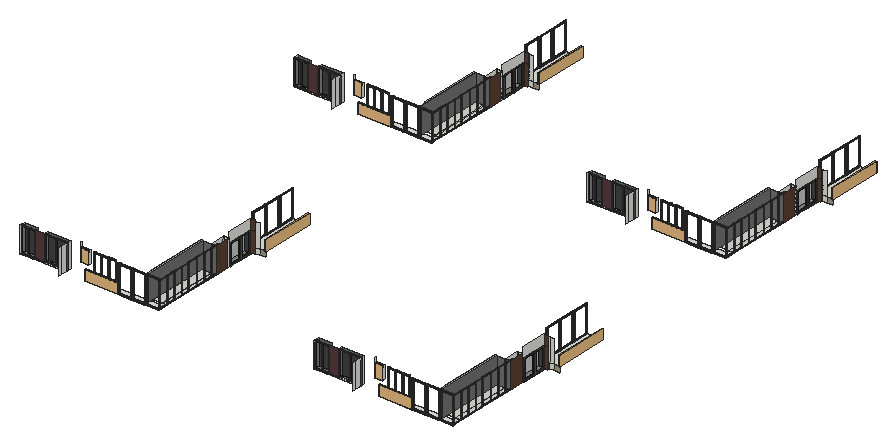
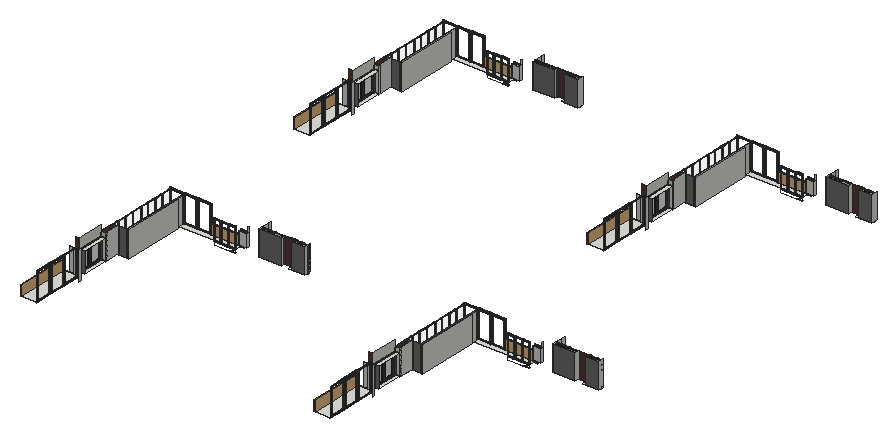
# SketchUp Ruby script. Lengths in inches.
U = 1.inch
M = Sketchup.active_model
def pt(a) = Geom::Point3d.new(a.map { |v| v * U })
def face(e, loops, mat)
  f = e.add_face(loops[0].map { |a| pt(a) })
  loops[1..].each { |l| e.add_face(l.map { |a| pt(a) }).erase! }
  f.material = f.back_material = mat if mat
  f
end
# faces: each face lists its corners as indices into pts; further lists are holes
def faces(e, pts, list, mat = nil) = list.each { |f| face(e, (f[0].is_a?(Array) ? f : [f]).map { |l| l.map { |i| pts[i] } }, mat) }
# xy, xz, yz: faces in a plane at the given z, y or x. An outline is a flat list of corners, or four numbers for a rectangle; further outlines are holes
def ring(l) = l.size == 4 ? [[l[0], l[1]], [l[2], l[1]], [l[2], l[3]], [l[0], l[3]]] : l.each_slice(2).to_a
def flat(e, list, mat, &to3) = list.each { |f| face(e, (f[0].is_a?(Array) ? f : [f]).map { |l| ring(l).map { |u, v| to3.(u, v) } }, mat) }
def xy(e, z, list, mat = nil) = flat(e, list, mat) { |x, y| [x, y, z] }
def xz(e, y, list, mat = nil) = flat(e, list, mat) { |x, z| [x, y, z] }
def yz(e, x, list, mat = nil) = flat(e, list, mat) { |y, z| [x, y, z] }
def lines(e, pts, list) = list.each { |a, b| e.add_line(pt(pts[a]), pt(pts[b])) }
# prism: a flat outline (further loops are holes) pulled along v
def prism(e, loops, v, mat = nil)
  f = face(e, loops, mat); d = Geom::Vector3d.new(v.map { |x| x * U })
  f.pushpull(f.normal.samedirection?(d) ? d.length : -d.length)
end
def box(e, o, s, mat = nil) = prism(e, [[o, [o[0] + s[0], o[1], o[2]], [o[0] + s[0], o[1] + s[1], o[2]], [o[0], o[1] + s[1], o[2]]]], [0, 0, s[2]], mat)
def at(x, y, z, deg = 0) = Geom::Transformation.translation(pt([x, y, z])) * Geom::Transformation.rotation(ORIGIN, Z_AXIS, deg.degrees)
def axes(o, x, y, z) = Geom::Transformation.new([*x, 0, *y, 0, *z, 0, *pt(o).to_a, 1])
def part(name) = M.definitions.add(name)
# library, detail: a bought-in or finely detailed component or shape, given as its bounding box
def library(name, o, s) = part(name).tap { |d| box(d.entities, o, s) }
def detail(e, o, s) = box(e.add_group.entities, o, s)
def put(e, d, t, mat = nil) = e.add_instance(d, t).tap { |i| i.material = mat if mat }
def group(e, t, mat = nil) = e.add_group.tap { |g| g.transformation = t; g.material = mat if mat }.entities
root = M.entities
M.materials.add("Glass_Tinted_Gray").color = [0, 0, 0]
M.materials["Glass_Tinted_Gray"].alpha = 0.125
M.materials.add("Glazing").color = [128, 128, 128]
M.materials["Glazing"].alpha = 0.05
M.materials.add("Powdercoating").color = [41, 44, 40]
M.materials.add("Wine2").color = [0, 0, 0]
M.materials["Wine2"].alpha = 0
M.materials.add("[0130_Gainsboro]").color = [39, 45, 50]
M.materials.add("[0135_DarkGray]").color = [81, 81, 81]
M.materials.add("[Color M05]").color = [114, 114, 114]
M.materials.add("[Color M06]").color = [86, 86, 86]
M.materials.add("[Concrete Tile]").color = [165, 155, 133]
M.materials.add("[Granite Brown]").color = [89, 59, 61]
M.materials.add("[Granite Brown]1").color = [89, 63, 50]
M.materials.add("[Mirror 02]").color = [229, 229, 229]
M.materials.add("[Terrazzo Light Blue]").color = [196, 214, 227]
c1 = part("Framed glazing panel")
xy(c1.entities,0,[[0,-0.98,43.07,0],[0,0,43.07,1.4]],"[0130_Gainsboro]")
xy(c1.entities,0.3,[[0.3,-1.43,42.77,-0.98]],"[0130_Gainsboro]")
xy(c1.entities,2.95,[[2.95,-1.43,40.12,-0.63],[2.95,-0.63,40.12,0],[2.95,0,40.12,0.64],[2.95,0.64,40.12,1.4]],"[0130_Gainsboro]")
xy(c1.entities,3.54,[[3.54,-0.63,39.53,0],[3.54,0,39.53,0.64]],"[0130_Gainsboro]")
xy(c1.entities,111.8125,[[3.54,-0.63,39.53,0],[3.54,0,39.53,0.64]],"[0130_Gainsboro]")
xy(c1.entities,112.4,[[2.95,-1.43,40.12,-0.63],[2.95,-0.63,40.12,0],[2.95,0,40.12,0.64],[2.95,0.64,40.12,1.4]],"[0130_Gainsboro]")
xy(c1.entities,115.05,[[0.3,-1.43,42.77,-0.98]],"[0130_Gainsboro]")
xy(c1.entities,115.35,[[0,-0.98,43.07,0],[0,0,43.07,1.4]],"[0130_Gainsboro]")
xz(c1.entities,-1.43,[[[0.3,0.3,42.77,115.05],[2.95,2.95,40.12,112.4]]],"[0130_Gainsboro]")
xz(c1.entities,-0.98,[[[0,0,43.07,115.35],[0.3,0.3,42.77,115.05]]],"[0130_Gainsboro]")
xz(c1.entities,-0.63,[[[2.95,2.95,40.12,112.4],[3.54,3.54,39.53,111.8125]]],"[0130_Gainsboro]")
xz(c1.entities,0,[[3.54,3.54,39.53,111.8125]],"Wine2")
xz(c1.entities,0,[[[0,0,43.07,115.35],[2.95,2.95,40.12,112.4]],[[2.95,2.95,40.12,112.4],[3.54,3.54,39.53,111.8125]]],"[0130_Gainsboro]")
xz(c1.entities,0.64,[[[2.95,2.95,40.12,112.4],[3.54,3.54,39.53,111.8125]]],"[0130_Gainsboro]")
xz(c1.entities,1.4,[[[0,0,43.07,115.35],[2.95,2.95,40.12,112.4]]],"[0130_Gainsboro]")
yz(c1.entities,0,[[-0.98,0,0,115.35],[0,0,1.4,115.35]],"[0130_Gainsboro]")
yz(c1.entities,0.3,[[-1.43,0.3,-0.98,115.05]],"[0130_Gainsboro]")
yz(c1.entities,2.95,[[-1.43,2.95,-0.63,112.4],[-0.63,2.95,0,112.4],[0,2.95,0.64,112.4],[0.64,2.95,1.4,112.4]],"[0130_Gainsboro]")
yz(c1.entities,3.54,[[-0.63,3.54,0,111.8125],[0,3.54,0.64,111.8125]],"[0130_Gainsboro]")
yz(c1.entities,39.53,[[-0.63,3.54,0,111.8125],[0,3.54,0.64,111.8125]],"[0130_Gainsboro]")
yz(c1.entities,40.12,[[-1.43,2.95,-0.63,112.4],[-0.63,2.95,0,112.4],[0,2.95,0.64,112.4],[0.64,2.95,1.4,112.4]],"[0130_Gainsboro]")
yz(c1.entities,42.77,[[-1.43,0.3,-0.98,115.05]],"[0130_Gainsboro]")
yz(c1.entities,43.07,[[-0.98,0,0,115.35],[0,0,1.4,115.35]],"[0130_Gainsboro]")
c2 = part("Glazed panel assembly")
put(c2.entities,c1,axes([90.57,1.43,0],[1.05148,0,0],[0,1,0],[0,0,1]))
put(c2.entities,c1,axes([0,1.43,0],[1.05148,0,0],[0,1,0],[0,0,1]))
put(c2.entities,c1,axes([45.29,1.43,0],[1.05148,0,0],[0,1,0],[0,0,1]))
c3 = library("Glass Railing",[0,0,0],[139.5,4.76,42])
c4 = part("PENTEK_RP Fineline 50S_Sliding_DoorCase_E1")
box(c4.entities,[0,0,0],[1.51,3.66,99.27],"[0135_DarkGray]")
c5 = part("PENTEK_RP Fineline 50S_SlidingDooe_Case_E2")
box(c5.entities,[0,0,0],[96.25,3.66,1.51],"[0135_DarkGray]")
c6 = part("pentek_RP Fineline 50S_SlidingDoor_Case")
put(c6.entities,c4,at(97.76,0,0))
put(c6.entities,c5,at(1.51,0,0))
put(c6.entities,c4,at(0,0,0))
put(c6.entities,c5,at(1.51,0,97.76))
c7 = part("PENTEK_RP Fineline 50S_SlidingDoor_GlazingBead_2")
box(c7.entities,[0,0,0],[0.56,0.59,94.39],"[0135_DarkGray]")
c8 = part("PENTEK_RP Fineline 50S_SlidingDoor_Glass")
box(c8.entities,[0,0,0],[46.58,0.16,94.39],"Glass_Tinted_Gray")
c9 = part("PENTEK_RP Fineline 50S_SlidingDoor_GlazingBead")
box(c9.entities,[0,0,0],[45.47,0.59,0.56],"[0135_DarkGray]")
c10 = part("PENTEK_RP Fineline 50S_SlidingDoor_Leaf_E1")
xy(c10.entities,0,[[0,0,0.93,1.97],[0.93,1.57,1.49,1.97]],"[0135_DarkGray]")
xy(c10.entities,96.25,[[0,0,0.93,0,0.93,1.57,1.49,1.57,1.49,1.97,0,1.97]],"[0135_DarkGray]")
xz(c10.entities,0,[[0,0,0.93,96.25]],"[0135_DarkGray]")
xz(c10.entities,1.57,[[0.93,0,1.49,95.32],[0.93,95.32,1.49,96.25]],"[0135_DarkGray]")
xz(c10.entities,1.97,[[0,0,1.49,96.25]],"[0135_DarkGray]")
yz(c10.entities,0,[[0,0,1.97,96.25]],"[0135_DarkGray]")
yz(c10.entities,0.93,[[0,0,1.57,0.93],[0,0.93,1.57,95.32],[0,95.32,1.57,96.25]],"[0135_DarkGray]")
yz(c10.entities,1.49,[[1.57,0,1.97,95.32],[1.57,95.32,1.97,96.25]],"[0135_DarkGray]")
c11 = part("PENTEK_RP Fineline 50S_SlidingDoor_Leaf_E2")
xy(c11.entities,0,[[0,0,0,1.57,0.56,1.57,0.56,1.97,46.02,1.97,46.02,1.57,46.58,1.57,46.58,0]],"[0135_DarkGray]")
xy(c11.entities,0.93,[[0,0,46.58,1.57]],"[0135_DarkGray]")
xy(c11.entities,1.49,[[0.56,1.57,46.02,1.97]],"[0135_DarkGray]")
xz(c11.entities,0,[[0,0,46.58,0.93]],"[0135_DarkGray]")
xz(c11.entities,1.57,[[0,0,0.56,0.93],[46.02,0,46.58,0.93],[0.56,0.93,46.02,1.49]],"[0135_DarkGray]")
xz(c11.entities,1.97,[[0.56,0,46.02,1.49]],"[0135_DarkGray]")
yz(c11.entities,0,[[0,0,1.57,0.93]],"[0135_DarkGray]")
yz(c11.entities,0.56,[[1.57,0,1.97,0.93],[1.57,0.93,1.97,1.49]],"[0135_DarkGray]")
yz(c11.entities,46.02,[[1.57,0,1.97,0.93],[1.57,0.93,1.97,1.49]],"[0135_DarkGray]")
yz(c11.entities,46.58,[[0,0,1.57,0.93]],"[0135_DarkGray]")
c12 = part("PENTEK_RP Fineline S_SlidingDoor_Leaf1")
put(c12.entities,c7,at(0.93,0,0.93))
put(c12.entities,c7,at(46.96,0,0.93))
put(c12.entities,c8,at(1.49,1.42,0.93))
put(c12.entities,c9,at(1.49,0,0.93))
put(c12.entities,c8,at(1.49,0.59,0.93),"[Terrazzo Light Blue]")
put(c12.entities,c10,at(0,0,0))
put(c12.entities,c10,axes([48.44,0,0],[-1,0,0],[0,1,0],[0,0,1]))
put(c12.entities,c11,axes([0.93,0,96.25],[1,0,0],[0,1,0],[0,0,-1]))
put(c12.entities,c11,at(0.93,0,0))
put(c12.entities,c9,at(1.49,0,94.77))
c13 = part("PENTEK_RP Fineline 50S_SlidingDoor_Leaf2")
put(c13.entities,c8,at(1.49,1.42,0.93))
put(c13.entities,c9,at(1.49,0,94.77))
put(c13.entities,c7,at(46.96,0,0.93))
put(c13.entities,c8,at(1.49,0.59,0.93),"[Mirror 02]")
put(c13.entities,c7,at(0.93,0,0.93))
put(c13.entities,c10,at(0,0,0))
put(c13.entities,c10,axes([48.44,0,0],[-1,0,0],[0,1,0],[0,0,1]))
put(c13.entities,c9,at(1.49,0,0.93))
put(c13.entities,c11,axes([0.93,0,96.25],[1,0,0],[0,1,0],[0,0,-1]))
put(c13.entities,c11,at(0.93,0,0))
c14 = part("PENTEK - Slimmest Steel Sliding Door / Window\#1")
put(c14.entities,c6,at(0,-1.88,-0.09))
put(c14.entities,c12,at(1.51,-2.27,1.42))
put(c14.entities,c13,at(49.32,-0.3,1.42))
c15 = part("Group\#15")
xy(c15.entities,0,[[0,-55.94,0.71,45.94]])
xy(c15.entities,0.2,[[0,-55.94,0.47,45.94],[0.47,45.94,0.71,46.42]])
xy(c15.entities,2.36,[[0.47,-55.94,0.71,46.42]])
xz(c15.entities,-55.94,[[0,0,0.71,0,0.71,2.36,0.47,2.36,0.47,0.2,0,0.2]])
xz(c15.entities,45.94,[[0,0,0.71,0.2]])
xz(c15.entities,46.42,[[0.47,0.2,0.71,2.36]])
yz(c15.entities,0,[[-55.94,0,45.94,0.2]])
yz(c15.entities,0.47,[[-55.94,0.2,46.42,2.36]])
yz(c15.entities,0.71,[[-55.94,0,45.94,0,45.94,0.2,46.42,0.2,46.42,2.36,-55.94,2.36]])
c16 = part("Group\#7")
xy(c16.entities,0,[[0,-59.09,0.71,45.94]])
xy(c16.entities,0.2,[[0,-59.09,0.47,45.94],[0.47,45.94,0.71,46.42]])
xy(c16.entities,2.36,[[0.47,-59.09,0.71,46.42]])
xz(c16.entities,-59.09,[[0,0,0.71,0,0.71,2.36,0.47,2.36,0.47,0.2,0,0.2]])
xz(c16.entities,45.94,[[0,0,0.71,0.2]])
xz(c16.entities,46.42,[[0.47,0.2,0.71,2.36]])
yz(c16.entities,0,[[-59.09,0,45.94,0.2]])
yz(c16.entities,0.47,[[-59.09,0.2,46.42,2.36]])
yz(c16.entities,0.71,[[-59.09,0,45.94,0,45.94,0.2,46.42,0.2,46.42,2.36,-59.09,2.36]])
c17 = part("Group\#16")
prism(c17.entities,[[[0.47,-56.18,0.2],[0,-56.18,0.2],[0,-56.18,0],[0.71,-56.18,0],[0.71,-56.18,2.36],[0.47,-56.18,2.36]]],[0,28.68,0])
c18 = part("Group\#10")
box(c18.entities,[-0.73,0,0],[27.99,0.55,102.05])
c19 = part("Group\#18")
xy(c19.entities,0,[[0.47,-56.18,0.47,-55.47,0,-55.47,0,-28.21,1.18,-28.21,1.18,-56.18]])
xy(c19.entities,0.2,[[0.71,-56.18,1.18,-28.21],[0,-55.47,0.47,-28.21],[0.47,-28.21,0.71,-27.74]])
xy(c19.entities,2.36,[[0.47,-56.18,0.71,-27.74]])
xz(c19.entities,-56.18,[[0.47,0,1.18,0,1.18,0.2,0.71,0.2,0.71,2.36,0.47,2.36]])
xz(c19.entities,-55.47,[[0,0,0.47,0.2]])
xz(c19.entities,-28.21,[[0,0,1.18,0.2]])
xz(c19.entities,-27.74,[[0.47,0.2,0.71,2.36]])
yz(c19.entities,0,[[-55.47,0,-28.21,0.2]])
yz(c19.entities,0.47,[[-56.18,0,-55.47,0.2],[-56.18,0.2,-27.74,2.36]])
yz(c19.entities,0.71,[[-56.18,0.2,-27.74,2.36]])
yz(c19.entities,1.18,[[-56.18,0,-28.21,0.2]])
c20 = part("Group\#34")
xy(c20.entities,0,[[-20.45,0,7.76,1.22]])
xy(c20.entities,0.06,[[-20.39,0.06,7.7,1.22]])
xy(c20.entities,0.47,[[-19.98,0,7.28,0.06]])
xy(c20.entities,101.89,[[-19.98,0,7.28,0.06]])
xy(c20.entities,102.3,[[-20.39,0.06,7.7,1.22]])
xy(c20.entities,102.36,[[-20.45,0,7.76,1.22]])
xz(c20.entities,0,[[[-20.45,0,7.76,102.36],[-19.98,0.47,7.28,101.89]]])
xz(c20.entities,0.06,[[[-20.39,0.06,7.7,102.3],[-19.98,0.47,7.28,101.89]]])
xz(c20.entities,1.22,[[[-20.45,0,7.76,102.36],[-20.39,0.06,7.7,102.3]]])
yz(c20.entities,-20.45,[[0,0,1.22,102.36]])
yz(c20.entities,-20.39,[[0.06,0.06,1.22,102.3]])
yz(c20.entities,-19.98,[[0,0.47,0.06,101.89]])
yz(c20.entities,7.28,[[0,0.47,0.06,101.89]])
yz(c20.entities,7.7,[[0.06,0.06,1.22,102.3]])
yz(c20.entities,7.76,[[0,0,1.22,102.36]])
c21 = part("Group\#6")
put(c21.entities,c15,axes([27.97,0,7.875],[1,0,0],[0,0,-1],[0,1,0]),"Powdercoating")
put(c21.entities,c16,axes([0.71,0,6.8],[-1,0,0],[0,0,-0.97687],[0,1,0]),"Powdercoating")
put(c21.entities,c17,axes([-27.5,0,-38.07],[0,0,-1],[-1,0,0],[0,1,0]),"Powdercoating")
put(c21.entities,c18,at(1.12,0.35,-38.39),"Glazing")
put(c21.entities,c19,axes([-27.5,0,63.35],[0,0,1],[-1,0,0],[0,1,0]),"Powdercoating")
put(c21.entities,c20,at(20.6875,1.0625,-38.54),"Powdercoating")
c22 = part("Sliding door assembly")
put(c22.entities,c21,at(-1.18,4.5,38.86))
g1 = group(c22.entities,at(84.74,4.5,38.86))
put(g1,c15,axes([-27.97,0,7.875],[-1,0,0],[0,0,-1],[0,1,0]),"Powdercoating")
put(g1,c16,axes([-0.71,0,6.8],[1,0,0],[0,0,-0.97687],[0,1,0]),"Powdercoating")
put(g1,c17,axes([27.5,0,-38.07],[0,0,-1],[1,0,0],[0,1,0]),"Powdercoating")
put(g1,c18,axes([-1.12,0.35,-38.39],[-1,0,0],[0,1,0],[0,0,1]),"Glazing")
put(g1,c19,axes([27.5,0,63.35],[0,0,1],[1,0,0],[0,1,0]),"Powdercoating")
put(g1,c20,axes([-20.6875,1.0625,-38.54],[-1,0,0],[0,1,0],[0,0,1]),"Powdercoating")
g2 = group(c22.entities,at(56.0625,4.5,38.86))
put(g2,c15,axes([-27.97,0,7.875],[-1,0,0],[0,0,-1],[0,1,0]),"Powdercoating")
put(g2,c17,axes([27.5,0,-38.07],[0,0,-1],[1,0,0],[0,1,0]),"Powdercoating")
put(g2,c18,axes([-1.12,0.35,-38.39],[-1,0,0],[0,1,0],[0,0,1]),"Glazing")
put(g2,c19,axes([27.5,0,63.35],[0,0,1],[1,0,0],[0,1,0]),"Powdercoating")
put(g2,c20,axes([-20.6875,1.0625,-38.54],[-1,0,0],[0,1,0],[0,0,1]),"Powdercoating")
g3 = group(g2,at(-0.71,0,6.8),"Powdercoating")
xy(g3,-45.34,[[0.47,0.2,0.71,2.36]])
xy(g3,-44.88,[[0,0,0.71,0.2]])
xy(g3,57.73,[[0,0,0.71,0,0.71,2.36,0.47,2.36,0.47,0.2,0,0.2]])
xz(g3,0,[[0,-44.88,0.71,57.73]])
xz(g3,0.2,[[0.47,-45.34,0.71,-44.88],[0,-44.88,0.47,57.73]])
xz(g3,2.36,[[0.47,-45.34,0.71,57.73]])
yz(g3,0,[[0,-44.88,0.2,57.73]])
yz(g3,0.47,[[0.2,-45.34,2.36,57.73]])
yz(g3,0.71,[[0.2,-45.34,2.36,-45.34,2.36,57.73,0,57.73,0,-44.88,0.2,-44.88]])
put(c22.entities,c21,axes([-33.94,4.5,38.86],[1.14218,0,0],[0,1,0],[0,0,1]))
c23 = part("sliding door")
put(c23.entities,c22,at(0,-4.5,-0.08))
c24 = library("Klein+raam",[128.36,12.7,0],[19.68,5.51,55.12])
xy(root,641.5625,[[611.65,1835.1875,632.49,1837.0625],[1829.84,1835.1875,1850.67,1837.0625],[611.65,3249.875,632.49,3251.75],[1829.84,3249.875,1850.67,3251.75]])
xy(root,641.875,[[611.65,1835.1875,632.49,1837.0625],[1829.84,1835.1875,1850.67,1837.0625],[611.65,3249.875,632.49,3251.75],[1829.84,3249.875,1850.67,3251.75]])
xy(root,648.6875,[[745.8,1795.6875,913.875,1795.6875,913.875,1833.5,890.875,1833.5,890.875,1822.9375,857.6875,1822.9375,857.6875,1812.1875,852.25,1812.1875,852.25,1822.9375,616.54,1822.9375,616.54,1799.9375,745.8,1799.9375],[1963.98,1795.6875,2132.0625,1795.6875,2132.0625,1833.5,2109.0625,1833.5,2109.0625,1822.9375,2075.875,1822.9375,2075.875,1812.1875,2070.4375,1812.1875,2070.4375,1822.9375,1834.73,1822.9375,1834.73,1799.9375,1963.98,1799.9375],[852.25,1812.1875,857.6875,1822.9375],[2070.4375,1812.1875,2075.875,1822.9375],[852.25,1822.9375,857.6875,1837.0625],
  [2070.4375,1822.9375,2075.875,1837.0625],[890.875,1833.5,913.875,1835.1875],[2109.0625,1833.5,2132.0625,1835.1875],[890.875,1835.1875,894.3125,2091.0625],[894.3125,1835.1875,913.875,2091.0625],
  [2109.0625,1835.1875,2112.5,2091.0625],[2112.5,1835.1875,2132.0625,2091.0625],[847.6875,1837.0625,852.25,2091.0625],[852.25,1837.0625,857.6875,2091.0625],[857.6875,1837.0625,890.875,2091.0625],
  [2065.875,1837.0625,2070.4375,2091.0625],[2070.4375,1837.0625,2075.875,2091.0625],[2075.875,1837.0625,2109.0625,2091.0625],[894.3125,2091.0625,913.875,2156.01],[2112.5,2091.0625,2132.0625,2156.01],
  [745.8,3210.375,913.875,3210.375,913.875,3248.1875,890.875,3248.1875,890.875,3237.625,857.6875,3237.625,857.6875,3226.875,852.25,3226.875,852.25,3237.625,616.54,3237.625,616.54,3214.625,745.8,3214.625],[1963.98,3210.375,2132.0625,3210.375,2132.0625,3248.1875,2109.0625,3248.1875,2109.0625,3237.625,2075.875,3237.625,2075.875,3226.875,2070.4375,3226.875,2070.4375,3237.625,1834.73,3237.625,1834.73,3214.625,1963.98,3214.625],[852.25,3226.875,857.6875,3237.625],[2070.4375,3226.875,2075.875,3237.625],[852.25,3237.625,857.6875,3251.75],
  [2070.4375,3237.625,2075.875,3251.75],[890.875,3248.1875,913.875,3249.875],[2109.0625,3248.1875,2132.0625,3249.875],[890.875,3249.875,894.3125,3505.75],[894.3125,3249.875,913.875,3505.75],
  [2109.0625,3249.875,2112.5,3505.75],[2112.5,3249.875,2132.0625,3505.75],[847.6875,3251.75,852.25,3505.75],[852.25,3251.75,857.6875,3505.75],[857.6875,3251.75,890.875,3505.75],
  [2065.875,3251.75,2070.4375,3505.75],[2070.4375,3251.75,2075.875,3505.75],[2075.875,3251.75,2109.0625,3505.75],[894.3125,3505.75,913.875,3570.7],[2112.5,3505.75,2132.0625,3570.7]])
xy(root,651.4375,[[333.89,1799.9375,401.8,1822.9375],[401.8,1799.9375,431.33,1806.5625],[431.33,1799.9375,523.04,1822.9375],[1552.08,1799.9375,1619.99,1822.9375],[1619.99,1799.9375,1649.52,1806.5625],
  [1649.52,1799.9375,1741.23,1822.9375],[333.89,3214.625,401.8,3237.625],[401.8,3214.625,431.33,3221.25],[431.33,3214.625,523.04,3237.625],[1552.08,3214.625,1619.99,3237.625],
  [1619.99,3214.625,1649.52,3221.25],[1649.52,3214.625,1741.23,3237.625]])
xy(root,653.36,[[890.875,2156.01,913.875,2266.33],[2109.0625,2156.01,2132.0625,2266.33],[890.875,3570.7,913.875,3681.01],[2109.0625,3570.7,2132.0625,3681.01]])
xy(root,660.0625,[[890.875,2295.875,954.6875,2518.89],[2109.0625,2295.875,2172.875,2518.89],[890.875,3710.5625,954.6875,3933.57],[2109.0625,3710.5625,2172.875,3933.57]])
xy(root,682.81,[[557.4,1837.0625,589.71,1845.8125],[1775.59,1837.0625,1807.9,1845.8125],[557.4,3251.75,589.71,3260.5],[1775.59,3251.75,1807.9,3260.5]])
xy(root,735.09,[[557.4,1837.0625,589.71,1845.8125],[1775.59,1837.0625,1807.9,1845.8125],[557.4,3251.75,589.71,3260.5],[1775.59,3251.75,1807.9,3260.5]])
xy(root,739.04,[[890.875,2156.01,913.875,2266.33],[2109.0625,2156.01,2132.0625,2266.33],[890.875,3570.7,913.875,3681.01],[2109.0625,3570.7,2132.0625,3681.01]])
xz(root,1806.5625,[[401.8,651.4375,431.33,651.4375,431.33,756,402.4,756,387.59,756.07,387.07,651.51],[1619.99,651.4375,1649.52,651.4375,1649.52,756,1620.59,756,1605.78,756.07,1605.26,651.51]],"[Granite Brown]")
xz(root,1812.1875,[[852.25,648.6875,857.6875,756],[2070.4375,648.6875,2075.875,756]])
xz(root,1822.9375,[[333.89,651.4375,387.07,651.4375,387.59,756,333.89,756],[431.33,651.4375,523.04,756],[1552.08,651.4375,1605.26,651.4375,1605.78,756,1552.08,756],[1649.52,651.4375,1741.23,756]],"[Color M05]")
xz(root,1835.1875,[[611.65,641.5625,632.49,641.875],[1829.84,641.5625,1850.67,641.875]])
xz(root,1835.1875,[[557.4,682.81,557.88,735.09],[1775.59,682.81,1776.07,735.09],[557.4,735.09,557.88,756],[1775.59,735.09,1776.07,756]],"[Granite Brown]")
xz(root,1845.8125,[[557.4,682.81,589.71,735.09],[1775.59,682.81,1807.9,735.09]])
xz(root,2091.0625,[[847.6875,648.6875,852.25,756],[852.25,648.6875,857.6875,756],[890.875,648.6875,894.3125,756],[2065.875,648.6875,2070.4375,756],[2070.4375,648.6875,2075.875,756],
  [2109.0625,648.6875,2112.5,756]])
xz(root,2091.0625,[[857.6875,648.6875,890.875,756],[894.3125,648.6875,913.875,756],[2075.875,648.6875,2109.0625,756],[2112.5,648.6875,2132.0625,756]],"[Color M05]")
xz(root,2156.01,[[894.3125,648.6875,913.875,653.36],[2112.5,648.6875,2132.0625,653.36],[890.875,653.36,894.3125,739.04],[894.3125,653.36,913.875,739.04],[2109.0625,653.36,2112.5,739.04],
  [2112.5,653.36,2132.0625,739.04],[894.3125,739.04,913.875,756],[2112.5,739.04,2132.0625,756]])
xz(root,2266.33,[[890.875,653.36,913.875,739.04],[2109.0625,653.36,2132.0625,739.04]],"[Color M05]")
xz(root,2266.33,[[913.875,653.36,930.75,739.04],[2132.0625,653.36,2148.9375,739.04],[913.875,739.04,930.75,779.36],[2132.0625,739.04,2148.9375,779.36]],"[Granite Brown]1")
xz(root,2295.875,[[913.875,637.75,930.75,660.0625],[2132.0625,637.75,2148.9375,660.0625],[890.875,660.0625,913.875,756],[913.875,660.0625,930.75,756],[2109.0625,660.0625,2132.0625,756],
  [2132.0625,660.0625,2148.9375,756]])
xz(root,2295.875,[[930.75,637.75,954.6875,660.0625],[2148.9375,637.75,2172.875,660.0625]],"[Concrete Tile]")
xz(root,3221.25,[[401.8,651.4375,431.33,651.4375,431.33,756,402.4,756,387.59,756.07,387.07,651.51],[1619.99,651.4375,1649.52,651.4375,1649.52,756,1620.59,756,1605.78,756.07,1605.26,651.51]],"[Granite Brown]")
xz(root,3226.875,[[852.25,648.6875,857.6875,756],[2070.4375,648.6875,2075.875,756]])
xz(root,3237.625,[[333.89,651.4375,387.07,651.4375,387.59,756,333.89,756],[431.33,651.4375,523.04,756],[1552.08,651.4375,1605.26,651.4375,1605.78,756,1552.08,756],[1649.52,651.4375,1741.23,756]],"[Color M05]")
xz(root,3249.875,[[611.65,641.5625,632.49,641.875],[1829.84,641.5625,1850.67,641.875]])
xz(root,3249.875,[[557.4,682.81,557.88,735.09],[1775.59,682.81,1776.07,735.09],[557.4,735.09,557.88,756],[1775.59,735.09,1776.07,756]],"[Granite Brown]")
xz(root,3260.5,[[557.4,682.81,589.71,735.09],[1775.59,682.81,1807.9,735.09]])
xz(root,3505.75,[[847.6875,648.6875,852.25,756],[852.25,648.6875,857.6875,756],[890.875,648.6875,894.3125,756],[2065.875,648.6875,2070.4375,756],[2070.4375,648.6875,2075.875,756],
  [2109.0625,648.6875,2112.5,756]])
xz(root,3505.75,[[857.6875,648.6875,890.875,756],[894.3125,648.6875,913.875,756],[2075.875,648.6875,2109.0625,756],[2112.5,648.6875,2132.0625,756]],"[Color M05]")
xz(root,3570.7,[[894.3125,648.6875,913.875,653.36],[2112.5,648.6875,2132.0625,653.36],[890.875,653.36,894.3125,739.04],[894.3125,653.36,913.875,739.04],[2109.0625,653.36,2112.5,739.04],
  [2112.5,653.36,2132.0625,739.04],[894.3125,739.04,913.875,756],[2112.5,739.04,2132.0625,756]])
xz(root,3681.01,[[890.875,653.36,913.875,739.04],[2109.0625,653.36,2132.0625,739.04]],"[Color M05]")
xz(root,3681.01,[[913.875,653.36,930.75,739.04],[2132.0625,653.36,2148.9375,739.04],[913.875,739.04,930.75,779.36],[2132.0625,739.04,2148.9375,779.36]],"[Granite Brown]1")
xz(root,3710.5625,[[913.875,637.75,930.75,660.0625],[2132.0625,637.75,2148.9375,660.0625],[890.875,660.0625,913.875,756],[913.875,660.0625,930.75,756],[2109.0625,660.0625,2132.0625,756],
  [2132.0625,660.0625,2148.9375,756]])
xz(root,3710.5625,[[930.75,637.75,954.6875,660.0625],[2148.9375,637.75,2172.875,660.0625]],"[Concrete Tile]")
yz(root,333.89,[[1799.9375,651.4375,1822.9375,756],[3214.625,651.4375,3237.625,756]])
yz(root,431.33,[[1806.5625,651.4375,1822.9375,756],[3221.25,651.4375,3237.625,756]])
yz(root,523.04,[[1763.25,651.4375,1822.9375,756],[3177.9375,651.4375,3237.625,756]])
yz(root,557.4,[[1835.1875,682.81,1845.8125,735.09],[3249.875,682.81,3260.5,735.09],[1835.1875,735.09,1837.0625,756],[3249.875,735.09,3251.75,756]])
yz(root,589.71,[[1837.0625,682.81,1845.8125,735.09],[3251.75,682.81,3260.5,735.09]])
yz(root,611.65,[[1835.1875,641.5625,1837.0625,641.875],[3249.875,641.5625,3251.75,641.875]])
yz(root,632.49,[[1835.1875,641.5625,1837.0625,641.875],[3249.875,641.5625,3251.75,641.875]])
yz(root,847.6875,[[1837.0625,648.6875,2091.0625,756],[3251.75,648.6875,3505.75,756]])
yz(root,852.25,[[1812.1875,648.6875,2091.0625,756],[3226.875,648.6875,3505.75,756]])
yz(root,857.6875,[[1812.1875,648.6875,2091.0625,756],[3226.875,648.6875,3505.75,756]],"[Color M05]")
yz(root,890.875,[[2290,637.75,2295.875,756],[3704.6875,637.75,3710.5625,756]])
yz(root,894.3125,[[2091.0625,648.6875,2148.83,756],[2148.83,648.6875,2156.01,756],[3505.75,648.6875,3563.51,756],[3563.51,648.6875,3570.7,756]])
yz(root,913.875,[[2148.83,648.6875,2156.01,756],[3563.51,648.6875,3570.7,756],[2156.01,739.04,2266.33,779.36],[3570.7,739.04,3681.01,779.36]])
yz(root,913.875,[[2091.0625,648.6875,2148.83,756],[3505.75,648.6875,3563.51,756]],"[Granite Brown]1")
yz(root,1552.08,[[1799.9375,651.4375,1822.9375,756],[3214.625,651.4375,3237.625,756]])
yz(root,1649.52,[[1806.5625,651.4375,1822.9375,756],[3221.25,651.4375,3237.625,756]])
yz(root,1741.23,[[1763.25,651.4375,1822.9375,756],[3177.9375,651.4375,3237.625,756]])
yz(root,1775.59,[[1835.1875,682.81,1845.8125,735.09],[3249.875,682.81,3260.5,735.09],[1835.1875,735.09,1837.0625,756],[3249.875,735.09,3251.75,756]])
yz(root,1807.9,[[1837.0625,682.81,1845.8125,735.09],[3251.75,682.81,3260.5,735.09]])
yz(root,1829.84,[[1835.1875,641.5625,1837.0625,641.875],[3249.875,641.5625,3251.75,641.875]])
yz(root,1850.67,[[1835.1875,641.5625,1837.0625,641.875],[3249.875,641.5625,3251.75,641.875]])
yz(root,2065.875,[[1837.0625,648.6875,2091.0625,756],[3251.75,648.6875,3505.75,756]])
yz(root,2070.4375,[[1812.1875,648.6875,2091.0625,756],[3226.875,648.6875,3505.75,756]])
yz(root,2075.875,[[1812.1875,648.6875,2091.0625,756],[3226.875,648.6875,3505.75,756]],"[Color M05]")
yz(root,2109.0625,[[2290,637.75,2295.875,756],[3704.6875,637.75,3710.5625,756]])
yz(root,2112.5,[[2091.0625,648.6875,2148.83,756],[2148.83,648.6875,2156.01,756],[3505.75,648.6875,3563.51,756],[3563.51,648.6875,3570.7,756]])
yz(root,2132.0625,[[2148.83,648.6875,2156.01,756],[3563.51,648.6875,3570.7,756],[2156.01,739.04,2266.33,779.36],[3570.7,739.04,3681.01,779.36]])
yz(root,2132.0625,[[2091.0625,648.6875,2148.83,756],[3505.75,648.6875,3563.51,756]],"[Granite Brown]1")
p = [[1829.84,1835.1875,641.5625],[1829.84,1835.1875,641.125],[1850.67,1835.1875,641.5625],[1850.67,1835.1875,641.125],[1919.77,1835.1875,641.5625],[1919.77,1835.1875,739.6875],
  [1919.77,1835.1875,641.125],[1829.84,1835.1875,739.6875],[1829.84,1835.1875,641.875],[1829.84,1835.1875,639.0625],[1850.67,1835.1875,639.0625],[1919.77,1835.1875,639.0625],
  [1741.23,1778.3125,651.4375],[1741.23,1778.3125,756],[611.65,1835.1875,639.0625],[632.49,1835.1875,639.0625],[701.59,1835.1875,639.0625],[701.59,1835.1875,641.125],
  [611.65,1835.1875,641.125],[701.59,1835.1875,739.6875],[611.65,1835.1875,739.6875],[611.65,1835.1875,641.875],[632.49,1835.1875,641.5625],[632.49,1835.1875,641.125],
  [611.65,1835.1875,641.5625],[701.59,1835.1875,641.5625],[523.04,1778.3125,651.4375],[523.04,1778.3125,756],[1741.23,3193,651.4375],[1741.23,3193,756],
  [1829.84,3249.875,641.125],[1829.84,3249.875,639.0625],[1919.77,3249.875,639.0625],[1919.77,3249.875,641.125],[1919.77,3249.875,739.6875],[1829.84,3249.875,739.6875],
  [1850.67,3249.875,639.0625],[1829.84,3249.875,641.875],[1919.77,3249.875,641.5625],[1850.67,3249.875,641.5625],[1850.67,3249.875,641.125],[1829.84,3249.875,641.5625],
  [611.65,3249.875,639.0625],[632.49,3249.875,639.0625],[701.59,3249.875,639.0625],[701.59,3249.875,641.125],[701.59,3249.875,739.6875],[611.65,3249.875,739.6875],
  [611.65,3249.875,641.125],[611.65,3249.875,641.5625],[611.65,3249.875,641.875],[701.59,3249.875,641.5625],[632.49,3249.875,641.5625],[632.49,3249.875,641.125],
  [523.04,3193,651.4375],[523.04,3193,756]]
lines(root,p,[[0,1],[2,3],[4,5],[6,4],[7,8],[5,7],[9,10],[1,3],[10,11],[1,9],[11,6],[12,13],
  [14,15],[16,17],[18,14],[19,20],[20,21],[22,23],[18,23],[15,16],[24,18],[17,25],[25,19],[26,27],
  [28,29],[30,31],[32,33],[34,35],[31,36],[35,37],[38,34],[39,40],[41,30],[33,38],[30,40],[36,32],
  [42,43],[44,45],[46,47],[48,42],[49,48],[47,50],[51,46],[52,53],[43,44],[45,51],[48,53],[54,55]])
put(root,c2,axes([1960.88,1795.6875,645.73],[1.25999,0,0],[0,1,0],[0,0,1]))
put(root,c2,axes([742.69,1795.6875,645.73],[1.25999,0,0],[0,1,0],[0,0,1]))
put(root,c2,axes([1960.88,3210.375,645.73],[1.25999,0,0],[0,1,0],[0,0,1]))
put(root,c2,axes([742.69,3210.375,645.73],[1.25999,0,0],[0,1,0],[0,0,1]))
put(root,c3,at(1821.78,1795.6875,646.04))
put(root,c3,at(603.59,1795.6875,646.04))
put(root,c3,at(1821.78,3210.375,646.04))
put(root,c3,at(603.59,3210.375,646.04))
put(root,c14,axes([1552.08,1806.83,648.45],[0.55914,0,0],[0,0.88,0],[0,0,1.08438]))
put(root,c14,axes([333.89,1806.83,648.45],[0.55914,0,0],[0,0.88,0],[0,0,1.08438]))
put(root,c14,axes([1552.08,3221.52,648.45],[0.55914,0,0],[0,0.88,0],[0,0,1.08438]))
put(root,c14,axes([333.89,3221.52,648.45],[0.55914,0,0],[0,0.88,0],[0,0,1.08438]))
put(root,c23,axes([2132.0625,1839.88,648.6875],[0,1.302,0],[-1,0,0],[0,0,1.03877]))
put(root,c23,axes([913.875,1839.88,648.6875],[0,1.302,0],[-1,0,0],[0,0,1.03877]))
put(root,c23,axes([2132.0625,3254.56,648.6875],[0,1.302,0],[-1,0,0],[0,0,1.03877]))
put(root,c23,axes([913.875,3254.56,648.6875],[0,1.302,0],[-1,0,0],[0,0,1.03877]))
put(root,c23,axes([2131,1993.48,649.42],[0,1.302,0],[-1,0,0],[0,0,1.03877]))
put(root,c23,axes([912.8125,1993.48,649.42],[0,1.302,0],[-1,0,0],[0,0,1.03877]))
put(root,c23,axes([2131,3408.17,649.42],[0,1.302,0],[-1,0,0],[0,0,1.03877]))
put(root,c23,axes([912.8125,3408.17,649.42],[0,1.302,0],[-1,0,0],[0,0,1.03877]))
put(root,c14,axes([2131.3,2158.32,650.8],[0,1.12181,0],[-2.51374,0,0],[0,0,0.87918]))
put(root,c14,axes([913.11,2158.32,650.8],[0,1.12181,0],[-2.51374,0,0],[0,0,0.87918]))
put(root,c14,axes([2131.3,3573.01,650.8],[0,1.12181,0],[-2.51374,0,0],[0,0,0.87918]))
put(root,c14,axes([913.11,3573.01,650.8],[0,1.12181,0],[-2.51374,0,0],[0,0,0.87918]))
put(root,c14,axes([1649.52,1808.21,651.53],[0.92473,0,0],[0,0.88,0],[0,0,1.054]))
put(root,c14,axes([431.33,1808.21,651.53],[0.92473,0,0],[0,0.88,0],[0,0,1.054]))
put(root,c14,axes([1649.52,3222.9,651.53],[0.92473,0,0],[0,0.88,0],[0,0,1.054]))
put(root,c14,axes([431.33,3222.9,651.53],[0.92473,0,0],[0,0.88,0],[0,0,1.054]))
put(root,c2,axes([1829.4375,1835.1875,653.1875],[0.6649,0,0],[0,0.61,0],[0,0,0.74986]),"[Color M06]")
put(root,c2,axes([611.25,1835.1875,653.1875],[0.6649,0,0],[0,0.61,0],[0,0,0.74986]),"[Color M06]")
put(root,c2,axes([1829.4375,3249.875,653.1875],[0.6649,0,0],[0,0.61,0],[0,0,0.74986]),"[Color M06]")
put(root,c2,axes([611.25,3249.875,653.1875],[0.6649,0,0],[0,0.61,0],[0,0,0.74986]),"[Color M06]")
put(root,c3,axes([2174.88,2295.6875,660.0625],[0,1.6,0],[-1,0,0],[0,0,1]))
put(root,c3,axes([956.7,2295.6875,660.0625],[0,1.6,0],[-1,0,0],[0,0,1]))
put(root,c3,axes([2174.88,3710.375,660.0625],[0,1.6,0],[-1,0,0],[0,0,1]))
put(root,c3,axes([956.7,3710.375,660.0625],[0,1.6,0],[-1,0,0],[0,0,1]))
put(root,c2,axes([2108.26,2309.55,660.0625],[0,1.54079,0],[-1,0,0],[0,0,1]))
put(root,c2,axes([890.08,2309.55,660.0625],[0,1.54079,0],[-1,0,0],[0,0,1]))
put(root,c2,axes([2108.26,3724.24,660.0625],[0,1.54079,0],[-1,0,0],[0,0,1]))
put(root,c2,axes([890.08,3724.24,660.0625],[0,1.54079,0],[-1,0,0],[0,0,1]))
put(root,c24,axes([1572.84,1824.68,682.81],[1.58777,0,0],[0,0.68,0],[0,0,0.99202]))
put(root,c24,axes([354.65,1824.68,682.81],[1.58777,0,0],[0,0.68,0],[0,0,0.99202]))
put(root,c24,axes([1572.84,3239.37,682.81],[1.58777,0,0],[0,0.68,0],[0,0,0.99202]))
put(root,c24,axes([354.65,3239.37,682.81],[1.58777,0,0],[0,0.68,0],[0,0,0.99202]))
